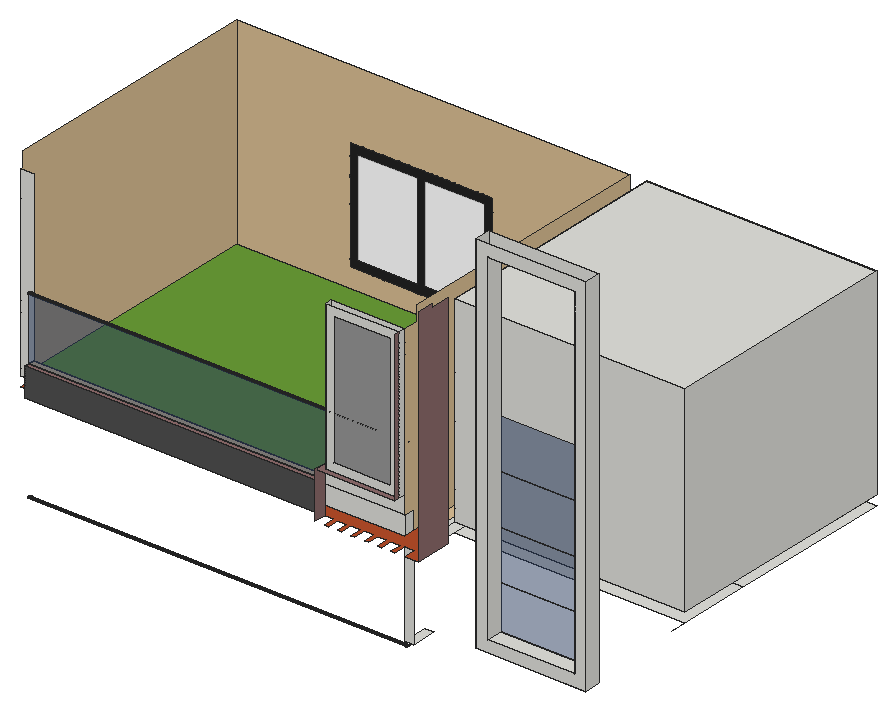
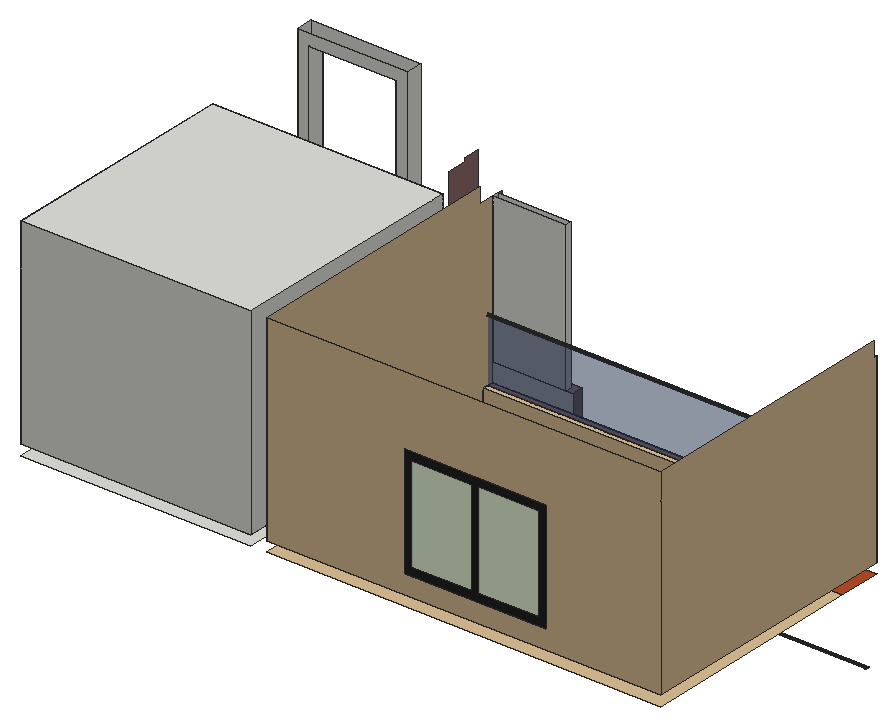
# SketchUp Ruby script. Lengths in inches.
U = 1.inch
M = Sketchup.active_model
def pt(a) = Geom::Point3d.new(a.map { |v| v * U })
def face(e, loops, mat)
  f = e.add_face(loops[0].map { |a| pt(a) })
  loops[1..].each { |l| e.add_face(l.map { |a| pt(a) }).erase! }
  f.material = f.back_material = mat if mat
  f
end
# faces: each face lists its corners as indices into pts; further lists are holes
def faces(e, pts, list, mat = nil) = list.each { |f| face(e, (f[0].is_a?(Array) ? f : [f]).map { |l| l.map { |i| pts[i] } }, mat) }
# xy, xz, yz: faces in a plane at the given z, y or x. An outline is a flat list of corners, or four numbers for a rectangle; further outlines are holes
def ring(l) = l.size == 4 ? [[l[0], l[1]], [l[2], l[1]], [l[2], l[3]], [l[0], l[3]]] : l.each_slice(2).to_a
def flat(e, list, mat, &to3) = list.each { |f| face(e, (f[0].is_a?(Array) ? f : [f]).map { |l| ring(l).map { |u, v| to3.(u, v) } }, mat) }
def xy(e, z, list, mat = nil) = flat(e, list, mat) { |x, y| [x, y, z] }
def xz(e, y, list, mat = nil) = flat(e, list, mat) { |x, z| [x, y, z] }
def yz(e, x, list, mat = nil) = flat(e, list, mat) { |y, z| [x, y, z] }
def lines(e, pts, list) = list.each { |a, b| e.add_line(pt(pts[a]), pt(pts[b])) }
# prism: a flat outline (further loops are holes) pulled along v
def prism(e, loops, v, mat = nil)
  f = face(e, loops, mat); d = Geom::Vector3d.new(v.map { |x| x * U })
  f.pushpull(f.normal.samedirection?(d) ? d.length : -d.length)
end
def box(e, o, s, mat = nil) = prism(e, [[o, [o[0] + s[0], o[1], o[2]], [o[0] + s[0], o[1] + s[1], o[2]], [o[0], o[1] + s[1], o[2]]]], [0, 0, s[2]], mat)
def at(x, y, z, deg = 0) = Geom::Transformation.translation(pt([x, y, z])) * Geom::Transformation.rotation(ORIGIN, Z_AXIS, deg.degrees)
def axes(o, x, y, z) = Geom::Transformation.new([*x, 0, *y, 0, *z, 0, *pt(o).to_a, 1])
def part(name) = M.definitions.add(name)
# library, detail: a bought-in or finely detailed component or shape, given as its bounding box
def library(name, o, s) = part(name).tap { |d| box(d.entities, o, s) }
def detail(e, o, s) = box(e.add_group.entities, o, s)
def put(e, d, t, mat = nil) = e.add_instance(d, t).tap { |i| i.material = mat if mat }
def group(e, t, mat = nil) = e.add_group.tap { |g| g.transformation = t; g.material = mat if mat }.entities
root = M.entities
M.materials.add("[0033_NavajoWhite]").color = [221, 193, 150]
M.materials.add("[0119_RosyBrown]").color = [142, 108, 108]
M.materials.add("[0119_RosyBrown]2").color = [142, 108, 108]
M.materials.add("[0135_DarkGray]").color = [81, 81, 81]
M.materials.add("[0136_Charcoal]").color = [35, 35, 35]
M.materials.add("[Beadboard]").color = [181, 77, 41]
M.materials.add("[Diamond Stripes]").color = [153, 153, 153]
M.materials.add("[Grass Dark Green]").color = [106, 157, 55]
M.materials.add("[Translucent Glass Blue]").color = [47, 70, 112]
M.materials["[Translucent Glass Blue]"].alpha = 0.5
M.materials.add("[Translucent Resin Crush Gray]").color = [249, 249, 249]
M.materials["[Translucent Resin Crush Gray]"].alpha = 0.8
box(root,[2453.375,1252.62,1536],[828,864,720])
xy(root,1197,[[2393.375,1102.62,2427.51,1192.62]])
xy(root,1242,[[2627.375,1132.62,3023.375,1192.62]])
xy(root,1284,[[2669.375,1132.62,2981.375,1192.62]])
xy(root,1500,[[1250.35,1169.13,1242.59,1170.15,1235.35,1173.15,1229.14,1177.92,1224.37,1184.13,1221.375,1191.37,1220.35,1199.13,1221.375,1206.9,1224.37,1214.13,1229.14,1220.35,1235.35,1225.11,1242.59,1228.11,1250.35,1229.13,1258.12,1228.11,1265.35,1225.11,1271.57,1220.35,1276.33,1214.13,1279.33,1206.9,1280.35,1199.13,1279.33,1191.37,1276.33,1184.13,1271.57,1177.92,1265.35,1173.15,1258.12,1170.15],[2023.98,1178.63,2016.21,1179.65,2008.98,1182.65,2002.76,1187.42,1998,1193.63,1995,1200.87,1993.98,1208.63,1995,1216.4,1998,1223.63,2002.76,1229.85,2008.98,1234.61,2016.21,1237.61,2023.98,1238.63,2031.74,1237.61,2038.98,1234.61,2045.19,1229.85,2049.96,1223.63,2052.95,1216.4,2053.98,1208.63,2052.95,1200.87,2049.96,1193.63,2045.19,1187.42,2038.98,1182.65,2031.74,1179.65],[2393.375,1192.62,2417.375,1516.62],[2417.375,1192.62,2453.375,1516.62],[2453.375,1252.62,3281.375,1516.62],
  [2453.375,1516.62,3281.375,2116.62],[1183.98,1837.44,1176.21,1838.47,1168.98,1841.46,1162.76,1846.23,1158,1852.44,1155,1859.68,1153.98,1867.44,1155,1875.21,1158,1882.44,1162.76,1888.66,1168.98,1893.43,1176.21,1896.42,1183.98,1897.44,1191.74,1896.42,1198.98,1893.43,1205.19,1888.66,1209.96,1882.44,1212.95,1875.21,1213.98,1867.44,1212.95,1859.68,1209.96,1852.44,1205.19,1846.23,1198.98,1841.46,1191.74,1838.47],[2023.98,1837.44,2016.21,1838.47,2008.98,1841.46,2002.76,1846.23,1998,1852.44,1995,1859.68,1993.98,1867.44,1995,1875.21,1998,1882.44,2002.76,1888.66,2008.98,1893.43,2016.21,1896.42,2023.98,1897.44,2031.74,1896.42,2038.98,1893.43,2045.19,1888.66,2049.96,1882.44,2052.95,1875.21,2053.98,1867.44,2052.95,1859.68,2049.96,1852.44,2045.19,1846.23,2038.98,1841.46,2031.74,1838.47]])
xy(root,1500,[[[977.375,1300.62,2393.375,2116.62],[2023.98,1837.44,2031.74,1838.47,2038.98,1841.46,2045.19,1846.23,2049.96,1852.44,2052.95,1859.68,2053.98,1867.44,2052.95,1875.21,2049.96,1882.44,2045.19,1888.66,2038.98,1893.43,2031.74,1896.42,2023.98,1897.44,2016.21,1896.42,2008.98,1893.43,2002.76,1888.66,1998,1882.44,1995,1875.21,1993.98,1867.44,1995,1859.68,1998,1852.44,2002.76,1846.23,2008.98,1841.46,2016.21,1838.47],[1183.98,1837.44,1191.74,1838.47,1198.98,1841.46,1205.19,1846.23,1209.96,1852.44,1212.95,1859.68,1213.98,1867.44,1212.95,1875.21,1209.96,1882.44,1205.19,1888.66,1198.98,1893.43,1191.74,1896.42,1183.98,1897.44,1176.21,1896.42,1168.98,1893.43,1162.76,1888.66,1158,1882.44,1155,1875.21,1153.98,1867.44,1155,1859.68,1158,1852.44,1162.76,1846.23,1168.98,1841.46,1176.21,1838.47]]],"[0033_NavajoWhite]")
xy(root,1500,[[[2139.51,1060.62,2139.51,1102.62,1025.375,1102.62,1025.375,1144.62,977.375,1144.62,977.375,1300.62,2393.375,1300.62,2393.375,1192.62,2477.375,1192.62,2477.375,1060.62,2427.51,1060.62,2427.51,1102.62,2393.375,1102.62,2393.375,1060.62,2379.51,1060.62,2379.51,1102.62,2345.375,1102.62,2345.375,1060.62,2331.51,1060.62,2331.51,1102.62,2297.375,1102.62,2297.375,1060.62,2283.51,1060.62,2283.51,1102.62,2249.375,1102.62,2249.375,1060.62,2235.51,1060.62,2235.51,1102.62,2201.375,1102.62,2201.375,1060.62,2187.51,1060.62,2187.51,1102.62,2153.375,1102.62,2153.375,1060.62],[1250.35,1169.13,1258.12,1170.15,1265.35,1173.15,1271.57,1177.92,1276.33,1184.13,1279.33,1191.37,1280.35,1199.13,1279.33,1206.9,1276.33,1214.13,1271.57,1220.35,1265.35,1225.11,1258.12,1228.11,1250.35,1229.13,1242.59,1228.11,1235.35,1225.11,1229.14,1220.35,1224.37,1214.13,1221.375,1206.9,1220.35,1199.13,1221.375,1191.37,1224.37,1184.13,1229.14,1177.92,1235.35,1173.15,1242.59,1170.15],[2023.98,1178.63,2031.74,1179.65,2038.98,1182.65,2045.19,1187.42,2049.96,1193.63,2052.95,1200.87,2053.98,1208.63,2052.95,1216.4,2049.96,1223.63,2045.19,1229.85,2038.98,1234.61,2031.74,1237.61,2023.98,1238.63,2016.21,1237.61,2008.98,1234.61,2002.76,1229.85,1998,1223.63,1995,1216.4,1993.98,1208.63,1995,1200.87,1998,1193.63,2002.76,1187.42,2008.98,1182.65,2016.21,1179.65]]],"[Beadboard]")
xy(root,1536,[[977.375,1144.62,2393.375,2116.62]],"[Grass Dark Green]")
xy(root,1602,[[1025.375,1123.62,2393.375,1144.62]],"[0033_NavajoWhite]")
xy(root,1602,[[1025.375,1102.62,2393.375,1123.62]],"[0119_RosyBrown]2")
xy(root,1668,[[2129.375,1078.62,2393.375,1102.62]])
xy(root,1668,[[2105.375,1060.62,2393.375,1060.62,2393.375,1078.62,2129.375,1078.62,2129.375,1102.62,2105.375,1102.62]],"[0119_RosyBrown]")
xz(root,1078.62,[[[2129.375,1668,2393.375,2203],[2159.375,1698,2363.375,2173]]])
xz(root,1078.62,[[2159.375,1698,2363.375,2173]],"[Diamond Stripes]")
xz(root,1102.62,[[2393.375,1197,2427.51,1500],[2105.375,1536,2393.375,1602],[2105.375,1602,2393.375,1668],[2129.375,1668,2393.375,2203]])
xz(root,1102.62,[[1025.375,1500,2105.375,1602]],"[0135_DarkGray]")
xz(root,1123.62,[[1025.375,1826,2393.375,1830]])
xz(root,1123.62,[[1025.375,1602,2393.375,1826]],"[Translucent Glass Blue]")
xz(root,1132.62,[[[2627.375,1242,3023.375,2562],[2669.375,1284,2981.375,2520]]])
xz(root,1144.62,[[977.375,1536,1025.375,2203]])
xz(root,1144.62,[[1025.375,1536,2393.375,1602]],"[0033_NavajoWhite]")
xz(root,1192.62,[[[2627.375,1242,3023.375,2562],[2669.375,1284,2981.375,2520]],[2393.375,1500,2477.375,1536]])
xz(root,1192.62,[[2669.375,1284,2981.375,1440],[2669.375,1440,2981.375,1620],[2669.375,1620,2981.375,1800],[2669.375,1800,2981.375,1980]],"[Translucent Glass Blue]")
xz(root,2116.62,[[[977.375,1536,2393.375,2256],[1385.74,1603.25,1902.43,2007.31]]],"[0033_NavajoWhite]")
xz(root,2116.62,[[[1385.74,1603.25,1902.43,2007.31],[1656.09,1633.25,1872.43,1977.31],[1415.74,1633.25,1632.09,1977.31]]],"[0136_Charcoal]")
xz(root,2116.62,[[1415.74,1633.25,1632.09,1977.31],[1656.09,1633.25,1872.43,1977.31]],"[Translucent Resin Crush Gray]")
yz(root,977.375,[[1144.62,1536,2116.62,1536,2116.62,2256,1156.62,2256,1156.62,2203,1144.62,2203]],"[0033_NavajoWhite]")
yz(root,1025.375,[[1102.62,1536,1144.62,1602],[1123.62,1826,1122.58,1826.14,1121.62,1826.54,1120.79,1827.17,1120.15,1828,1119.75,1828.96,1119.62,1830,1119.75,1831.04,1120.15,1832,1120.79,1832.83,1121.62,1833.46,1122.58,1833.86,1123.62,1834,1124.65,1833.86,1125.62,1833.46,1126.45,1832.83,1127.08,1832,1127.48,1831.04,1127.62,1830,1127.48,1828.96,1127.08,1828,1126.45,1827.17,1125.62,1826.54,1124.65,1826.14]])
yz(root,2105.375,[[1060.62,1500,1102.62,1668]],"[0119_RosyBrown]2")
yz(root,2129.375,[[1078.62,1668,1102.62,2203]])
yz(root,2393.375,[[1102.62,1536,1144.62,1602],[1078.62,1668,1102.62,2203]])
yz(root,2393.375,[[[1144.62,1536,1144.62,1602,1102.62,1602,1102.62,2203,1156.62,2203,1156.62,2256,2116.62,2256,2116.62,1536],[1123.62,1826,1124.65,1826.14,1125.62,1826.54,1126.45,1827.17,1127.08,1828,1127.48,1828.96,1127.62,1830,1127.48,1831.04,1127.08,1832,1126.45,1832.83,1125.62,1833.46,1124.65,1833.86,1123.62,1834,1122.58,1833.86,1121.62,1833.46,1120.79,1832.83,1120.15,1832,1119.75,1831.04,1119.62,1830,1119.75,1828.96,1120.15,1828,1120.79,1827.17,1121.62,1826.54,1122.58,1826.14]]],"[0033_NavajoWhite]")
yz(root,2393.375,[[1060.62,1668,1078.62,2203]],"[0119_RosyBrown]")
yz(root,2477.375,[[1060.62,1500,1192.62,1500,1192.62,2292,1120.62,2292,1120.62,2305.2,1060.62,2305.2]],"[0119_RosyBrown]")
yz(root,2627.375,[[1132.62,1242,1192.62,2562]])
yz(root,2669.375,[[1132.62,1284,1192.62,2520]])
yz(root,2981.375,[[1132.62,1284,1192.62,2520]])
yz(root,3023.375,[[1132.62,1242,1192.62,2562]])
p = [[1025.375,1119.62,1170],[1025.375,1119.75,1168.96],[2393.375,1119.75,1168.96],[2393.375,1119.62,1170],[1025.375,1127.48,1168.96],[1025.375,1127.62,1170],
  [2393.375,1127.62,1170],[2393.375,1127.48,1168.96],[1025.375,1119.75,1171.04],[2393.375,1119.75,1171.04],[1025.375,1127.48,1171.04],[2393.375,1127.48,1171.04],
  [1025.375,1120.15,1172],[2393.375,1120.15,1172],[1025.375,1127.08,1172],[2393.375,1127.08,1172],[1025.375,1120.79,1172.83],[2393.375,1120.79,1172.83],
  [1025.375,1126.45,1172.83],[2393.375,1126.45,1172.83],[1025.375,1121.62,1173.46],[2393.375,1121.62,1173.46],[1025.375,1125.62,1173.46],[2393.375,1125.62,1173.46],
  [1025.375,1122.58,1173.86],[2393.375,1122.58,1173.86],[1025.375,1124.65,1173.86],[2393.375,1124.65,1173.86],[1025.375,1123.62,1174],[2393.375,1123.62,1174],
  [1025.375,1122.58,1826.14],[1025.375,1123.62,1826],[2393.375,1123.62,1826],[2393.375,1122.58,1826.14],[1025.375,1124.65,1826.14],[2393.375,1124.65,1826.14],
  [1025.375,1121.62,1826.54],[2393.375,1121.62,1826.54],[1025.375,1125.62,1826.54],[2393.375,1125.62,1826.54],[1025.375,1120.79,1827.17],[2393.375,1120.79,1827.17],
  [1025.375,1126.45,1827.17],[2393.375,1126.45,1827.17],[1025.375,1120.15,1828],[2393.375,1120.15,1828],[1025.375,1127.08,1828],[2393.375,1127.08,1828],
  [1025.375,1119.75,1828.96],[2393.375,1119.75,1828.96],[1025.375,1127.48,1828.96],[2393.375,1127.48,1828.96],[1025.375,1119.62,1830],[2393.375,1119.62,1830],
  [1025.375,1127.62,1830],[2393.375,1127.62,1830],[1025.375,1119.75,1831.04],[2393.375,1119.75,1831.04],[1025.375,1127.48,1831.04],[2393.375,1127.48,1831.04],
  [1025.375,1120.15,1832],[2393.375,1120.15,1832],[1025.375,1127.08,1832],[2393.375,1127.08,1832],[1025.375,1120.79,1832.83],[2393.375,1120.79,1832.83],
  [1025.375,1126.45,1832.83],[2393.375,1126.45,1832.83],[1025.375,1121.62,1833.46],[2393.375,1121.62,1833.46],[1025.375,1125.62,1833.46],[2393.375,1125.62,1833.46],
  [3281.375,1252.62,1500],[3281.375,1192.62,1500],[2129.375,1078.62,1668],[2129.375,1078.62,1665.25]]
faces(root,p,[[0,1,2,3],[4,5,6,7],[8,0,3,9],[5,10,11,6],[12,8,9,13],[10,14,15,11],[16,12,13,17],[14,18,19,15],
  [20,16,17,21],[18,22,23,19],[24,20,21,25],[22,26,27,23],[28,24,25,29],[26,28,29,27],[30,31,32,33],[31,34,35,32],
  [36,30,33,37],[34,38,39,35],[40,36,37,41],[38,42,43,39],[44,40,41,45],[42,46,47,43],[48,44,45,49],[46,50,51,47],
  [52,48,49,53],[50,54,55,51],[56,52,53,57],[54,58,59,55],[60,56,57,61],[58,62,63,59],[64,60,61,65],[62,66,67,63],
  [68,64,65,69],[66,70,71,67]],"[0136_Charcoal]")
lines(root,p,[[72,73],[74,75]])
